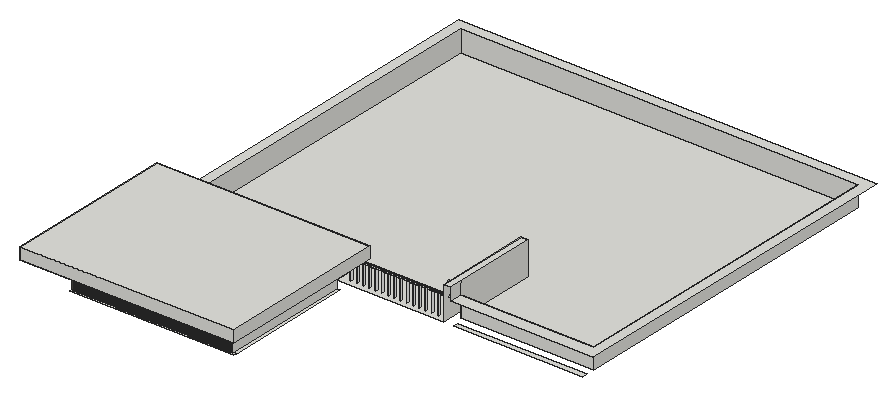
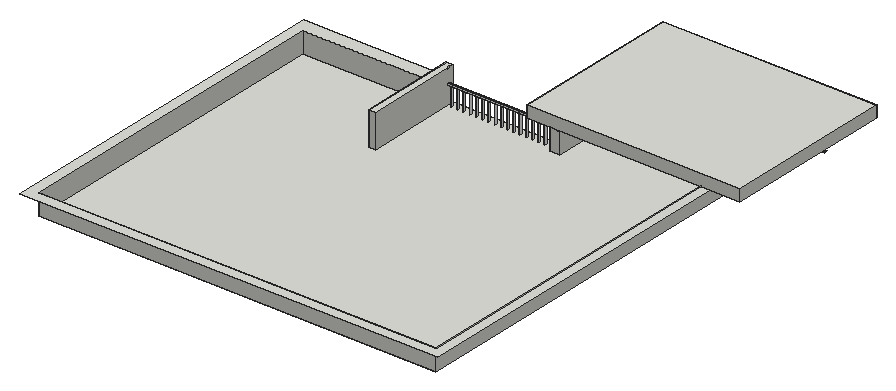
# SketchUp Ruby script. Lengths in inches.
U = 1.inch
M = Sketchup.active_model
def pt(a) = Geom::Point3d.new(a.map { |v| v * U })
def face(e, loops, mat)
  f = e.add_face(loops[0].map { |a| pt(a) })
  loops[1..].each { |l| e.add_face(l.map { |a| pt(a) }).erase! }
  f.material = f.back_material = mat if mat
  f
end
# faces: each face lists its corners as indices into pts; further lists are holes
def faces(e, pts, list, mat = nil) = list.each { |f| face(e, (f[0].is_a?(Array) ? f : [f]).map { |l| l.map { |i| pts[i] } }, mat) }
# xy, xz, yz: faces in a plane at the given z, y or x. An outline is a flat list of corners, or four numbers for a rectangle; further outlines are holes
def ring(l) = l.size == 4 ? [[l[0], l[1]], [l[2], l[1]], [l[2], l[3]], [l[0], l[3]]] : l.each_slice(2).to_a
def flat(e, list, mat, &to3) = list.each { |f| face(e, (f[0].is_a?(Array) ? f : [f]).map { |l| ring(l).map { |u, v| to3.(u, v) } }, mat) }
def xy(e, z, list, mat = nil) = flat(e, list, mat) { |x, y| [x, y, z] }
def xz(e, y, list, mat = nil) = flat(e, list, mat) { |x, z| [x, y, z] }
def yz(e, x, list, mat = nil) = flat(e, list, mat) { |y, z| [x, y, z] }
def lines(e, pts, list) = list.each { |a, b| e.add_line(pt(pts[a]), pt(pts[b])) }
# prism: a flat outline (further loops are holes) pulled along v
def prism(e, loops, v, mat = nil)
  f = face(e, loops, mat); d = Geom::Vector3d.new(v.map { |x| x * U })
  f.pushpull(f.normal.samedirection?(d) ? d.length : -d.length)
end
def box(e, o, s, mat = nil) = prism(e, [[o, [o[0] + s[0], o[1], o[2]], [o[0] + s[0], o[1] + s[1], o[2]], [o[0], o[1] + s[1], o[2]]]], [0, 0, s[2]], mat)
def at(x, y, z, deg = 0) = Geom::Transformation.translation(pt([x, y, z])) * Geom::Transformation.rotation(ORIGIN, Z_AXIS, deg.degrees)
def axes(o, x, y, z) = Geom::Transformation.new([*x, 0, *y, 0, *z, 0, *pt(o).to_a, 1])
def part(name) = M.definitions.add(name)
# library, detail: a bought-in or finely detailed component or shape, given as its bounding box
def library(name, o, s) = part(name).tap { |d| box(d.entities, o, s) }
def detail(e, o, s) = box(e.add_group.entities, o, s)
def put(e, d, t, mat = nil) = e.add_instance(d, t).tap { |i| i.material = mat if mat }
def group(e, t, mat = nil) = e.add_group.tap { |g| g.transformation = t; g.material = mat if mat }.entities
root = M.entities
M.materials.add("CALACATA").color = [248, 248, 247]
M.materials.add("Wood_Planks_01_1K").color = [69, 67, 63]
xy(root,253,[[25.35,188.73,166.52,188.73,166.52,191.73,163.52,191.73,163.52,190.73,162.02,190.73,162.02,191.73,161.24,191.73,161.24,190.73,159.74,190.73,159.74,191.73,158.96,191.73,158.96,190.73,157.46,190.73,157.46,191.73,156.69,191.73,156.69,190.73,155.19,190.73,155.19,191.73,154.41,191.73,154.41,190.73,152.91,190.73,152.91,191.73,152.13,191.73,152.13,190.73,150.63,190.73,150.63,191.73,149.85,191.73,149.85,190.73,148.35,190.73,148.35,191.73,147.57,191.73,147.57,190.73,146.07,190.73,146.07,191.73,145.3,191.73,145.3,190.73,143.8,190.73,143.8,191.73,143.02,191.73,143.02,190.73,141.52,190.73,141.52,191.73,140.74,191.73,140.74,190.73,139.24,190.73,139.24,191.73,138.46,191.73,138.46,190.73,136.96,190.73,136.96,191.73,136.19,191.73,136.19,190.73,134.69,190.73,134.69,191.73,133.91,191.73,133.91,190.73,132.41,190.73,132.41,191.73,131.63,191.73,131.63,190.73,130.13,190.73,130.13,191.73,129.35,191.73,129.35,190.73,127.85,190.73,127.85,191.73,127.07,191.73,127.07,190.73,125.57,190.73,125.57,191.73,124.8,191.73,124.8,190.73,123.3,190.73,123.3,191.73,122.52,191.73,122.52,190.73,121.02,190.73,121.02,191.73,120.24,191.73,120.24,190.73,118.74,190.73,118.74,191.73,117.96,191.73,117.96,190.73,116.46,190.73,116.46,191.73,115.69,191.73,115.69,190.73,114.19,190.73,114.19,191.73,113.41,191.73,113.41,190.73,111.91,190.73,111.91,191.73,111.13,191.73,111.13,190.73,109.63,190.73,109.63,191.73,108.85,191.73,108.85,190.73,107.35,190.73,107.35,191.73,106.57,191.73,106.57,190.73,105.07,190.73,105.07,191.73,104.3,191.73,104.3,190.73,102.8,190.73,102.8,191.73,102.02,191.73,102.02,190.73,100.52,190.73,100.52,191.73,99.74,191.73,99.74,190.73,98.24,190.73,98.24,191.73,97.46,191.73,97.46,190.73,95.96,190.73,95.96,191.73,95.19,191.73,95.19,190.73,93.69,190.73,93.69,191.73,92.91,191.73,92.91,190.73,91.41,190.73,91.41,191.73,90.63,191.73,90.63,190.73,89.13,190.73,89.13,191.73,88.35,191.73,88.35,190.73,86.85,190.73,86.85,191.73,86.07,191.73,86.07,190.73,84.57,190.73,84.57,191.73,83.8,191.73,83.8,190.73,82.3,190.73,82.3,191.73,81.52,191.73,81.52,190.73,80.02,190.73,80.02,191.73,79.24,191.73,79.24,190.73,77.74,190.73,77.74,191.73,76.96,191.73,76.96,190.73,75.46,190.73,75.46,191.73,74.6875,191.73,74.6875,190.73,73.1875,190.73,73.1875,191.73,72.41,191.73,72.41,190.73,70.91,190.73,70.91,191.73,70.13,191.73,70.13,190.73,68.63,190.73,68.63,191.73,67.85,191.73,67.85,190.73,66.35,190.73,66.35,191.73,65.57,191.73,65.57,190.73,64.07,190.73,64.07,191.73,63.3,191.73,63.3,190.73,61.8,190.73,61.8,191.73,61.02,191.73,61.02,190.73,59.52,190.73,59.52,191.73,58.74,191.73,58.74,190.73,57.24,190.73,57.24,191.73,56.46,191.73,56.46,190.73,54.96,190.73,54.96,191.73,54.1875,191.73,54.1875,190.73,52.6875,190.73,52.6875,191.73,51.91,191.73,51.91,190.73,50.41,190.73,50.41,191.73,49.63,191.73,49.63,190.73,48.13,190.73,48.13,191.73,47.35,191.73,47.35,190.73,45.85,190.73,45.85,191.73,45.07,191.73,45.07,190.73,43.57,190.73,43.57,191.73,42.8,191.73,42.8,190.73,41.3,190.73,41.3,191.73,40.52,191.73,40.52,190.73,39.02,190.73,39.02,191.73,38.24,191.73,38.24,190.73,36.74,190.73,36.74,191.73,35.96,191.73,35.96,190.73,34.46,190.73,34.46,191.73,33.6875,191.73,33.6875,190.73,32.1875,190.73,32.1875,191.73,31.41,191.73,31.41,190.73,29.91,190.73,29.91,191.73,29.13,191.73,29.13,190.73,27.63,190.73,27.63,191.73,26.85,191.73,26.85,190.73,25.35,190.73],[163.52,191.73,166.52,302.73]])
xy(root,260,[[33.77,200.73,154.52,200.73,154.52,313.98,163.52,313.98,163.52,302.73,255.75,302.73,255.75,386.34,261.75,386.34,261.75,314.04,375.75,314.04,375.75,598.49,33.77,598.49],[264.75,302.73,375.75,307.15]])
xy(root,276.6,[[171.56,308.07,171.79,308.07,171.79,309.5],[163.52,308.125,170.98,309.5],[171.79,308.125,171.79,309.5,255.75,309.5,255.75,308.125,253.19,308.125,253.19,308.63,252.38,308.63,252.38,308.125,247.76,308.125,247.76,308.69,246.95,308.69,246.95,308.125,242.34,308.125,242.34,308.75,241.52,308.75,241.52,308.125,236.91,308.125,236.91,308.81,236.1,308.81,236.1,308.125,231.48,308.125,231.48,308.87,230.67,308.87,230.67,308.125,226.06,308.125,226.06,308.92,225.24,308.92,225.24,308.125,220.63,308.125,220.63,308.98,219.82,308.98,219.82,308.125,215.2,308.125,215.2,309.04,214.39,309.04,214.39,308.125,209.78,308.125,209.78,309.1,208.96,309.1,208.96,308.125,204.35,308.125,204.35,309.15,203.54,309.15,203.54,308.125,198.92,308.125,198.92,309.21,198.11,309.21,198.11,308.125,193.5,308.125,193.5,309.27,192.68,309.27,192.68,308.125,188.07,308.125,188.07,309.33,187.26,309.33,187.26,308.125,182.64,308.125,182.64,309.39,181.83,309.39,181.83,308.125,177.22,308.125,177.22,309.44,176.4,309.44,176.4,308.125],[176.4,308.125,177.22,309.44],[181.83,308.125,182.64,309.39],
  [187.26,308.125,188.07,309.33],[192.68,308.125,193.5,309.27],[198.11,308.125,198.92,309.21],[203.54,308.125,204.35,309.15],[208.96,308.125,209.78,309.1],
  [214.39,308.125,215.2,309.04],[219.82,308.125,220.63,308.98],[225.24,308.125,226.06,308.92],[230.67,308.125,231.48,308.87],[236.1,308.125,236.91,308.81],
  [241.52,308.125,242.34,308.75],[246.95,308.125,247.76,308.69],[252.38,308.125,253.19,308.63]],"CALACATA")
xy(root,277.75,[[163.52,308.125,255.75,309.5]],"CALACATA")
xy(root,278,[[25.35,190.73,26.85,190.73,26.85,191.73,27.63,191.73,27.63,190.73,29.13,190.73,29.13,191.73,29.91,191.73,29.91,190.73,31.41,190.73,31.41,191.73,32.1875,191.73,32.1875,190.73,33.6875,190.73,33.6875,191.73,34.46,191.73,34.46,190.73,35.96,190.73,35.96,191.73,36.74,191.73,36.74,190.73,38.24,190.73,38.24,191.73,39.02,191.73,39.02,190.73,40.52,190.73,40.52,191.73,41.3,191.73,41.3,190.73,42.8,190.73,42.8,191.73,43.57,191.73,43.57,190.73,45.07,190.73,45.07,191.73,45.85,191.73,45.85,190.73,47.35,190.73,47.35,191.73,48.13,191.73,48.13,190.73,49.63,190.73,49.63,191.73,50.41,191.73,50.41,190.73,51.91,190.73,51.91,191.73,52.6875,191.73,52.6875,190.73,54.1875,190.73,54.1875,191.73,54.96,191.73,54.96,190.73,56.46,190.73,56.46,191.73,57.24,191.73,57.24,190.73,58.74,190.73,58.74,191.73,59.52,191.73,59.52,190.73,61.02,190.73,61.02,191.73,61.8,191.73,61.8,190.73,63.3,190.73,63.3,191.73,64.07,191.73,64.07,190.73,65.57,190.73,65.57,191.73,66.35,191.73,66.35,190.73,67.85,190.73,67.85,191.73,68.63,191.73,68.63,190.73,70.13,190.73,70.13,191.73,70.91,191.73,70.91,190.73,72.41,190.73,72.41,191.73,73.1875,191.73,73.1875,190.73,74.6875,190.73,74.6875,191.73,75.46,191.73,75.46,190.73,76.96,190.73,76.96,191.73,77.74,191.73,77.74,190.73,79.24,190.73,79.24,191.73,80.02,191.73,80.02,190.73,81.52,190.73,81.52,191.73,82.3,191.73,82.3,190.73,83.8,190.73,83.8,191.73,84.57,191.73,84.57,190.73,86.07,190.73,86.07,191.73,86.85,191.73,86.85,190.73,88.35,190.73,88.35,191.73,89.13,191.73,89.13,190.73,90.63,190.73,90.63,191.73,91.41,191.73,91.41,190.73,92.91,190.73,92.91,191.73,93.69,191.73,93.69,190.73,95.19,190.73,95.19,191.73,95.96,191.73,95.96,190.73,97.46,190.73,97.46,191.73,98.24,191.73,98.24,190.73,99.74,190.73,99.74,191.73,100.52,191.73,100.52,190.73,102.02,190.73,102.02,191.73,102.8,191.73,102.8,190.73,104.3,190.73,104.3,191.73,105.07,191.73,105.07,190.73,106.57,190.73,106.57,191.73,107.35,191.73,107.35,190.73,108.85,190.73,108.85,191.73,109.63,191.73,109.63,190.73,111.13,190.73,111.13,191.73,111.91,191.73,111.91,190.73,113.41,190.73,113.41,191.73,114.19,191.73,114.19,190.73,115.69,190.73,115.69,191.73,116.46,191.73,116.46,190.73,117.96,190.73,117.96,191.73,118.74,191.73,118.74,190.73,120.24,190.73,120.24,191.73,121.02,191.73,121.02,190.73,122.52,190.73,122.52,191.73,123.3,191.73,123.3,190.73,124.8,190.73,124.8,191.73,125.57,191.73,125.57,190.73,127.07,190.73,127.07,191.73,127.85,191.73,127.85,190.73,129.35,190.73,129.35,191.73,130.13,191.73,130.13,190.73,131.63,190.73,131.63,191.73,132.41,191.73,132.41,190.73,133.91,190.73,133.91,191.73,134.69,191.73,134.69,190.73,136.19,190.73,136.19,191.73,136.96,191.73,136.96,190.73,138.46,190.73,138.46,191.73,139.24,191.73,139.24,190.73,140.74,190.73,140.74,191.73,141.52,191.73,141.52,190.73,143.02,190.73,143.02,191.73,143.8,191.73,143.8,190.73,145.3,190.73,145.3,191.73,146.07,191.73,146.07,190.73,147.57,190.73,147.57,191.73,148.35,191.73,148.35,190.73,149.85,190.73,149.85,191.73,150.63,191.73,150.63,190.73,152.13,190.73,152.13,191.73,152.91,191.73,152.91,190.73,154.41,190.73,154.41,191.73,155.19,191.73,155.19,190.73,156.69,190.73,156.69,191.73,157.46,191.73,157.46,190.73,158.96,190.73,158.96,191.73,159.74,191.73,159.74,190.73,161.24,190.73,161.24,191.73,162.02,191.73,162.02,190.73,163.52,190.73,163.52,313.98,154.52,313.98,154.52,200.73,25.35,200.73],[25.35,200.73,33.77,200.73,33.77,598.49,375.75,598.49,375.75,314.04,261.75,314.04,261.75,302.73,384.75,302.73,384.75,607.49,25.35,607.49]])
xy(root,288.73,[[255.75,302.73,261.75,386.34]])
xz(root,190.73,[[162.02,253,163.52,278]])
xz(root,190.73,[[25.35,253,26.85,278],[27.63,253,29.13,278],[29.91,253,31.41,278],[32.1875,253,33.6875,278],[34.46,253,35.96,278],
  [36.74,253,38.24,278],[39.02,253,40.52,278],[41.3,253,42.8,278],[43.57,253,45.07,278],[45.85,253,47.35,278],
  [48.13,253,49.63,278],[50.41,253,51.91,278],[52.6875,253,54.1875,278],[54.96,253,56.46,278],[57.24,253,58.74,278],
  [59.52,253,61.02,278],[61.8,253,63.3,278],[64.07,253,65.57,278],[66.35,253,67.85,278],[68.63,253,70.13,278],
  [70.91,253,72.41,278],[73.1875,253,74.6875,278],[75.46,253,76.96,278],[77.74,253,79.24,278],[80.02,253,81.52,278],
  [82.3,253,83.8,278],[84.57,253,86.07,278],[86.85,253,88.35,278],[89.13,253,90.63,278],[91.41,253,92.91,278],
  [93.69,253,95.19,278],[95.96,253,97.46,278],[98.24,253,99.74,278],[100.52,253,102.02,278],[102.8,253,104.3,278],
  [105.07,253,106.57,278],[107.35,253,108.85,278],[109.63,253,111.13,278],[111.91,253,113.41,278],[114.19,253,115.69,278],
  [116.46,253,117.96,278],[118.74,253,120.24,278],[121.02,253,122.52,278],[123.3,253,124.8,278],[125.57,253,127.07,278],
  [127.85,253,129.35,278],[130.13,253,131.63,278],[132.41,253,133.91,278],[134.69,253,136.19,278],[136.96,253,138.46,278],
  [139.24,253,140.74,278],[141.52,253,143.02,278],[143.8,253,145.3,278],[146.07,253,147.57,278],[148.35,253,149.85,278],
  [150.63,253,152.13,278],[152.91,253,154.41,278],[155.19,253,156.69,278],[157.46,253,158.96,278],[159.74,253,161.24,278]],"Wood_Planks_01_1K")
xz(root,191.73,[[26.85,253,27.63,278],[29.13,253,29.91,278],[31.41,253,32.1875,278],[33.6875,253,34.46,278],[35.96,253,36.74,278],
  [38.24,253,39.02,278],[40.52,253,41.3,278],[42.8,253,43.57,278],[45.07,253,45.85,278],[47.35,253,48.13,278],
  [49.63,253,50.41,278],[51.91,253,52.6875,278],[54.1875,253,54.96,278],[56.46,253,57.24,278],[58.74,253,59.52,278],
  [61.02,253,61.8,278],[63.3,253,64.07,278],[65.57,253,66.35,278],[67.85,253,68.63,278],[70.13,253,70.91,278],
  [72.41,253,73.1875,278],[74.6875,253,75.46,278],[76.96,253,77.74,278],[79.24,253,80.02,278],[81.52,253,82.3,278],
  [83.8,253,84.57,278],[86.07,253,86.85,278],[88.35,253,89.13,278],[90.63,253,91.41,278],[92.91,253,93.69,278],
  [95.19,253,95.96,278],[97.46,253,98.24,278],[99.74,253,100.52,278],[102.02,253,102.8,278],[104.3,253,105.07,278],
  [106.57,253,107.35,278],[108.85,253,109.63,278],[111.13,253,111.91,278],[113.41,253,114.19,278],[115.69,253,116.46,278],
  [117.96,253,118.74,278],[120.24,253,121.02,278],[122.52,253,123.3,278],[124.8,253,125.57,278],[127.07,253,127.85,278],
  [129.35,253,130.13,278],[131.63,253,132.41,278],[133.91,253,134.69,278],[136.19,253,136.96,278],[138.46,253,139.24,278],
  [140.74,253,141.52,278],[143.02,253,143.8,278],[145.3,253,146.07,278],[147.57,253,148.35,278],[149.85,253,150.63,278],
  [152.13,253,152.91,278],[154.41,253,155.19,278],[156.69,253,157.46,278],[158.96,253,159.74,278],[161.24,253,162.02,278]])
xz(root,200.73,[[25.35,260,33.77,278],[33.77,260,154.52,278]])
xz(root,307.26,[[252.38,260,253.19,276.6]],"CALACATA")
xz(root,307.32,[[246.95,260,247.76,276.6]],"CALACATA")
xz(root,307.375,[[241.52,260,242.34,276.6]],"CALACATA")
xz(root,307.43,[[236.1,260,236.91,276.6]],"CALACATA")
xz(root,307.49,[[230.67,260,231.48,276.6]],"CALACATA")
xz(root,307.55,[[225.24,260,226.06,276.6]],"CALACATA")
xz(root,307.61,[[219.82,260,220.63,276.6]],"CALACATA")
xz(root,307.66,[[214.39,260,215.2,276.6]],"CALACATA")
xz(root,307.72,[[208.96,260,209.78,276.6]],"CALACATA")
xz(root,307.78,[[203.54,260,204.35,276.6]],"CALACATA")
xz(root,307.84,[[198.11,260,198.92,276.6]],"CALACATA")
xz(root,307.9,[[192.68,260,193.5,276.6]],"CALACATA")
xz(root,307.95,[[187.26,260,188.07,276.6]],"CALACATA")
xz(root,308.01,[[181.83,260,182.64,276.6]],"CALACATA")
xz(root,308.07,[[176.4,260,177.22,276.6]],"CALACATA")
xz(root,308.125,[[170.98,260,171.79,260,171.79,276.6,255.75,276.6,255.75,277.75,163.52,277.75,163.52,276.6,170.98,276.6]],"CALACATA")
xz(root,308.63,[[252.38,260,253.19,276.6]],"CALACATA")
xz(root,308.69,[[246.95,260,247.76,276.6]],"CALACATA")
xz(root,308.75,[[241.52,260,242.34,276.6]],"CALACATA")
xz(root,308.81,[[236.1,260,236.91,276.6]],"CALACATA")
xz(root,308.87,[[230.67,260,231.48,276.6]],"CALACATA")
xz(root,308.92,[[225.24,260,226.06,276.6]],"CALACATA")
xz(root,308.98,[[219.82,260,220.63,276.6]],"CALACATA")
xz(root,309.04,[[214.39,260,215.2,276.6]],"CALACATA")
xz(root,309.1,[[208.96,260,209.78,276.6]],"CALACATA")
xz(root,309.15,[[203.54,260,204.35,276.6]],"CALACATA")
xz(root,309.21,[[198.11,260,198.92,276.6]],"CALACATA")
xz(root,309.27,[[192.68,260,193.5,276.6]],"CALACATA")
xz(root,309.33,[[187.26,260,188.07,276.6]],"CALACATA")
xz(root,309.39,[[181.83,260,182.64,276.6]],"CALACATA")
xz(root,309.44,[[176.4,260,177.22,276.6]],"CALACATA")
xz(root,309.5,[[170.98,260,170.98,276.6,163.52,276.6,163.52,277.75,255.75,277.75,255.75,276.6,171.79,276.6,171.79,260]],"CALACATA")
xz(root,313.98,[[154.52,260,163.52,278]])
xz(root,314.04,[[261.75,260,375.75,278]])
xz(root,386.34,[[255.75,260,261.75,288.73]])
xz(root,598.49,[[33.77,260,375.75,278]])
yz(root,26.85,[[190.73,253,191.73,278]])
yz(root,27.63,[[190.73,253,191.73,278]])
yz(root,29.13,[[190.73,253,191.73,278]])
yz(root,29.91,[[190.73,253,191.73,278]])
yz(root,31.41,[[190.73,253,191.73,278]])
yz(root,32.1875,[[190.73,253,191.73,278]])
yz(root,33.6875,[[190.73,253,191.73,278]])
yz(root,33.77,[[200.73,260,598.49,278]])
yz(root,34.46,[[190.73,253,191.73,278]])
yz(root,35.96,[[190.73,253,191.73,278]])
yz(root,36.74,[[190.73,253,191.73,278]])
yz(root,38.24,[[190.73,253,191.73,278]])
yz(root,39.02,[[190.73,253,191.73,278]])
yz(root,40.52,[[190.73,253,191.73,278]])
yz(root,41.3,[[190.73,253,191.73,278]])
yz(root,42.8,[[190.73,253,191.73,278]])
yz(root,43.57,[[190.73,253,191.73,278]])
yz(root,45.07,[[190.73,253,191.73,278]])
yz(root,45.85,[[190.73,253,191.73,278]])
yz(root,47.35,[[190.73,253,191.73,278]])
yz(root,48.13,[[190.73,253,191.73,278]])
yz(root,49.63,[[190.73,253,191.73,278]])
yz(root,50.41,[[190.73,253,191.73,278]])
yz(root,51.91,[[190.73,253,191.73,278]])
yz(root,52.6875,[[190.73,253,191.73,278]])
yz(root,54.1875,[[190.73,253,191.73,278]])
yz(root,54.96,[[190.73,253,191.73,278]])
yz(root,56.46,[[190.73,253,191.73,278]])
yz(root,57.24,[[190.73,253,191.73,278]])
yz(root,58.74,[[190.73,253,191.73,278]])
yz(root,59.52,[[190.73,253,191.73,278]])
yz(root,61.02,[[190.73,253,191.73,278]])
yz(root,61.8,[[190.73,253,191.73,278]])
yz(root,63.3,[[190.73,253,191.73,278]])
yz(root,64.07,[[190.73,253,191.73,278]])
yz(root,65.57,[[190.73,253,191.73,278]])
yz(root,66.35,[[190.73,253,191.73,278]])
yz(root,67.85,[[190.73,253,191.73,278]])
yz(root,68.63,[[190.73,253,191.73,278]])
yz(root,70.13,[[190.73,253,191.73,278]])
yz(root,70.91,[[190.73,253,191.73,278]])
yz(root,72.41,[[190.73,253,191.73,278]])
yz(root,73.1875,[[190.73,253,191.73,278]])
yz(root,74.6875,[[190.73,253,191.73,278]])
yz(root,75.46,[[190.73,253,191.73,278]])
yz(root,76.96,[[190.73,253,191.73,278]])
yz(root,77.74,[[190.73,253,191.73,278]])
yz(root,79.24,[[190.73,253,191.73,278]])
yz(root,80.02,[[190.73,253,191.73,278]])
yz(root,81.52,[[190.73,253,191.73,278]])
yz(root,82.3,[[190.73,253,191.73,278]])
yz(root,83.8,[[190.73,253,191.73,278]])
yz(root,84.57,[[190.73,253,191.73,278]])
yz(root,86.07,[[190.73,253,191.73,278]])
yz(root,86.85,[[190.73,253,191.73,278]])
yz(root,88.35,[[190.73,253,191.73,278]])
yz(root,89.13,[[190.73,253,191.73,278]])
yz(root,90.63,[[190.73,253,191.73,278]])
yz(root,91.41,[[190.73,253,191.73,278]])
yz(root,92.91,[[190.73,253,191.73,278]])
yz(root,93.69,[[190.73,253,191.73,278]])
yz(root,95.19,[[190.73,253,191.73,278]])
yz(root,95.96,[[190.73,253,191.73,278]])
yz(root,97.46,[[190.73,253,191.73,278]])
yz(root,98.24,[[190.73,253,191.73,278]])
yz(root,99.74,[[190.73,253,191.73,278]])
yz(root,100.52,[[190.73,253,191.73,278]])
yz(root,102.02,[[190.73,253,191.73,278]])
yz(root,102.8,[[190.73,253,191.73,278]])
yz(root,104.3,[[190.73,253,191.73,278]])
yz(root,105.07,[[190.73,253,191.73,278]])
yz(root,106.57,[[190.73,253,191.73,278]])
yz(root,107.35,[[190.73,253,191.73,278]])
yz(root,108.85,[[190.73,253,191.73,278]])
yz(root,109.63,[[190.73,253,191.73,278]])
yz(root,111.13,[[190.73,253,191.73,278]])
yz(root,111.91,[[190.73,253,191.73,278]])
yz(root,113.41,[[190.73,253,191.73,278]])
yz(root,114.19,[[190.73,253,191.73,278]])
yz(root,115.69,[[190.73,253,191.73,278]])
yz(root,116.46,[[190.73,253,191.73,278]])
yz(root,117.96,[[190.73,253,191.73,278]])
yz(root,118.74,[[190.73,253,191.73,278]])
yz(root,120.24,[[190.73,253,191.73,278]])
yz(root,121.02,[[190.73,253,191.73,278]])
yz(root,122.52,[[190.73,253,191.73,278]])
yz(root,123.3,[[190.73,253,191.73,278]])
yz(root,124.8,[[190.73,253,191.73,278]])
yz(root,125.57,[[190.73,253,191.73,278]])
yz(root,127.07,[[190.73,253,191.73,278]])
yz(root,127.85,[[190.73,253,191.73,278]])
yz(root,129.35,[[190.73,253,191.73,278]])
yz(root,130.13,[[190.73,253,191.73,278]])
yz(root,131.63,[[190.73,253,191.73,278]])
yz(root,132.41,[[190.73,253,191.73,278]])
yz(root,133.91,[[190.73,253,191.73,278]])
yz(root,134.69,[[190.73,253,191.73,278]])
yz(root,136.19,[[190.73,253,191.73,278]])
yz(root,136.96,[[190.73,253,191.73,278]])
yz(root,138.46,[[190.73,253,191.73,278]])
yz(root,139.24,[[190.73,253,191.73,278]])
yz(root,140.74,[[190.73,253,191.73,278]])
yz(root,141.52,[[190.73,253,191.73,278]])
yz(root,143.02,[[190.73,253,191.73,278]])
yz(root,143.8,[[190.73,253,191.73,278]])
yz(root,145.3,[[190.73,253,191.73,278]])
yz(root,146.07,[[190.73,253,191.73,278]])
yz(root,147.57,[[190.73,253,191.73,278]])
yz(root,148.35,[[190.73,253,191.73,278]])
yz(root,149.85,[[190.73,253,191.73,278]])
yz(root,150.63,[[190.73,253,191.73,278]])
yz(root,152.13,[[190.73,253,191.73,278]])
yz(root,152.91,[[190.73,253,191.73,278]])
yz(root,154.41,[[190.73,253,191.73,278]])
yz(root,154.52,[[200.73,260,313.98,278]])
yz(root,155.19,[[190.73,253,191.73,278]])
yz(root,156.69,[[190.73,253,191.73,278]])
yz(root,157.46,[[190.73,253,191.73,278]])
yz(root,158.96,[[190.73,253,191.73,278]])
yz(root,159.74,[[190.73,253,191.73,278]])
yz(root,161.24,[[190.73,253,191.73,278]])
yz(root,162.02,[[190.73,253,191.73,278]])
yz(root,163.52,[[190.73,253,302.73,253,302.73,260,313.98,260,313.98,278,190.73,278]])
yz(root,163.52,[[308.125,276.6,309.5,277.75]],"CALACATA")
yz(root,170.98,[[308.125,260,309.5,276.6]],"CALACATA")
yz(root,171.79,[[308.125,260,309.5,276.6]],"CALACATA")
yz(root,176.4,[[308.07,260,309.44,276.6]],"CALACATA")
yz(root,177.22,[[308.07,260,309.44,276.6]],"CALACATA")
yz(root,181.83,[[308.01,260,309.39,276.6]],"CALACATA")
yz(root,182.64,[[308.01,260,309.39,276.6]],"CALACATA")
yz(root,187.26,[[307.95,260,309.33,276.6]],"CALACATA")
yz(root,188.07,[[307.95,260,309.33,276.6]],"CALACATA")
yz(root,192.68,[[307.9,260,309.27,276.6]],"CALACATA")
yz(root,193.5,[[307.9,260,309.27,276.6]],"CALACATA")
yz(root,198.11,[[307.84,260,309.21,276.6]],"CALACATA")
yz(root,198.92,[[307.84,260,309.21,276.6]],"CALACATA")
yz(root,203.54,[[307.78,260,309.15,276.6]],"CALACATA")
yz(root,204.35,[[307.78,260,309.15,276.6]],"CALACATA")
yz(root,208.96,[[307.72,260,309.1,276.6]],"CALACATA")
yz(root,209.78,[[307.72,260,309.1,276.6]],"CALACATA")
yz(root,214.39,[[307.66,260,309.04,276.6]],"CALACATA")
yz(root,215.2,[[307.66,260,309.04,276.6]],"CALACATA")
yz(root,219.82,[[307.61,260,308.98,276.6]],"CALACATA")
yz(root,220.63,[[307.61,260,308.98,276.6]],"CALACATA")
yz(root,225.24,[[307.55,260,308.92,276.6]],"CALACATA")
yz(root,226.06,[[307.55,260,308.92,276.6]],"CALACATA")
yz(root,230.67,[[307.49,260,308.87,276.6]],"CALACATA")
yz(root,231.48,[[307.49,260,308.87,276.6]],"CALACATA")
yz(root,236.1,[[307.43,260,308.81,276.6]],"CALACATA")
yz(root,236.91,[[307.43,260,308.81,276.6]],"CALACATA")
yz(root,241.52,[[307.375,260,308.75,276.6]],"CALACATA")
yz(root,242.34,[[307.375,260,308.75,276.6]],"CALACATA")
yz(root,246.95,[[307.32,260,308.69,276.6]],"CALACATA")
yz(root,247.76,[[307.32,260,308.69,276.6]],"CALACATA")
yz(root,252.38,[[307.26,260,308.63,276.6]],"CALACATA")
yz(root,253.19,[[307.26,260,308.63,276.6]],"CALACATA")
yz(root,255.75,[[302.73,260,386.34,288.73]])
yz(root,255.75,[[308.125,276.6,309.5,277.75]],"CALACATA")
yz(root,261.75,[[314.04,260,386.34,288.73],[302.73,278,314.04,288.73]])
yz(root,375.75,[[314.04,260,598.49,278]])
p = [[255.52,308.85,289.72],[255.52,308.85,288.66],[255.75,307.15,288.66],[255.75,307.15,288.73],[255.75,307.15,289.72],[253.19,307.95,288.66],
  [255.52,307.95,288.66],[176.4,308.07,276.6],[171.79,308.07,276.6]]
faces(root,p,[[0,1,2,3,4]])
lines(root,p,[[5,6],[7,8]])
g1 = group(root,at(25.35,190.73,278))
box(g1,[-25.35,-24,0],[183.65,147.25,10])
